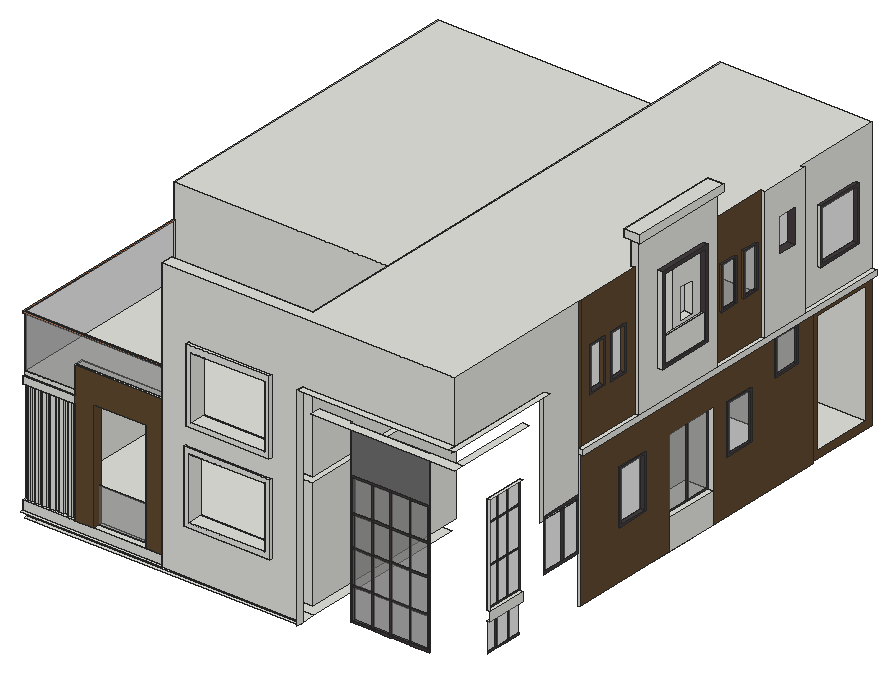
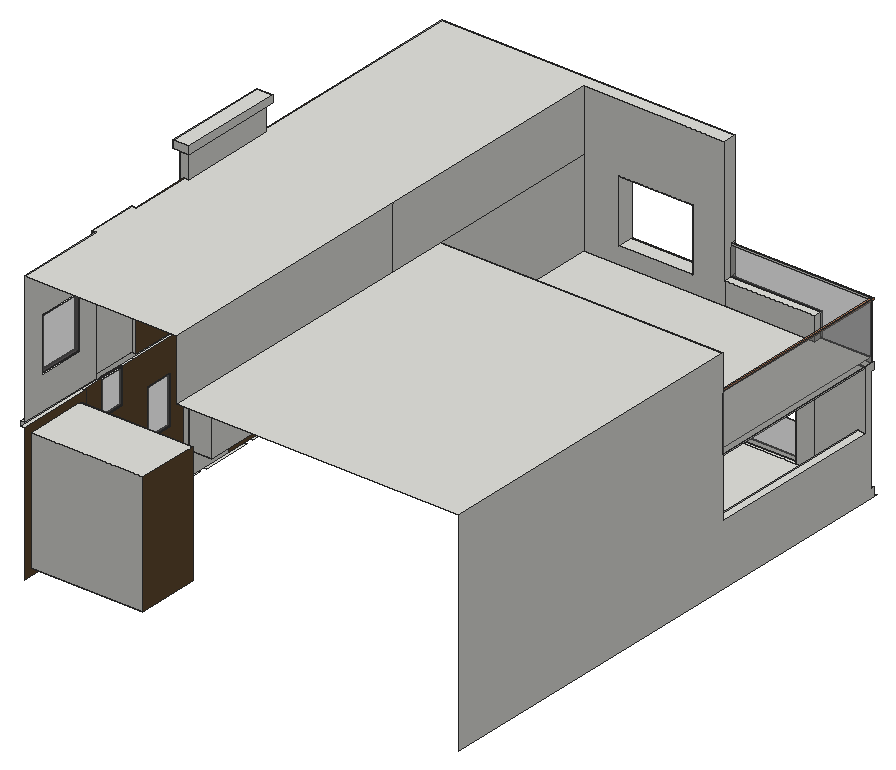
# SketchUp Ruby script. Lengths in inches.
U = 1.inch
M = Sketchup.active_model
def pt(a) = Geom::Point3d.new(a.map { |v| v * U })
def face(e, loops, mat)
  f = e.add_face(loops[0].map { |a| pt(a) })
  loops[1..].each { |l| e.add_face(l.map { |a| pt(a) }).erase! }
  f.material = f.back_material = mat if mat
  f
end
# faces: each face lists its corners as indices into pts; further lists are holes
def faces(e, pts, list, mat = nil) = list.each { |f| face(e, (f[0].is_a?(Array) ? f : [f]).map { |l| l.map { |i| pts[i] } }, mat) }
# xy, xz, yz: faces in a plane at the given z, y or x. An outline is a flat list of corners, or four numbers for a rectangle; further outlines are holes
def ring(l) = l.size == 4 ? [[l[0], l[1]], [l[2], l[1]], [l[2], l[3]], [l[0], l[3]]] : l.each_slice(2).to_a
def flat(e, list, mat, &to3) = list.each { |f| face(e, (f[0].is_a?(Array) ? f : [f]).map { |l| ring(l).map { |u, v| to3.(u, v) } }, mat) }
def xy(e, z, list, mat = nil) = flat(e, list, mat) { |x, y| [x, y, z] }
def xz(e, y, list, mat = nil) = flat(e, list, mat) { |x, z| [x, y, z] }
def yz(e, x, list, mat = nil) = flat(e, list, mat) { |y, z| [x, y, z] }
def lines(e, pts, list) = list.each { |a, b| e.add_line(pt(pts[a]), pt(pts[b])) }
# prism: a flat outline (further loops are holes) pulled along v
def prism(e, loops, v, mat = nil)
  f = face(e, loops, mat); d = Geom::Vector3d.new(v.map { |x| x * U })
  f.pushpull(f.normal.samedirection?(d) ? d.length : -d.length)
end
def box(e, o, s, mat = nil) = prism(e, [[o, [o[0] + s[0], o[1], o[2]], [o[0] + s[0], o[1] + s[1], o[2]], [o[0], o[1] + s[1], o[2]]]], [0, 0, s[2]], mat)
def at(x, y, z, deg = 0) = Geom::Transformation.translation(pt([x, y, z])) * Geom::Transformation.rotation(ORIGIN, Z_AXIS, deg.degrees)
def axes(o, x, y, z) = Geom::Transformation.new([*x, 0, *y, 0, *z, 0, *pt(o).to_a, 1])
def part(name) = M.definitions.add(name)
# library, detail: a bought-in or finely detailed component or shape, given as its bounding box
def library(name, o, s) = part(name).tap { |d| box(d.entities, o, s) }
def detail(e, o, s) = box(e.add_group.entities, o, s)
def put(e, d, t, mat = nil) = e.add_instance(d, t).tap { |i| i.material = mat if mat }
def group(e, t, mat = nil) = e.add_group.tap { |g| g.transformation = t; g.material = mat if mat }.entities
root = M.entities
M.materials.add("Niraj_Hair_Dark").color = [109, 109, 109]
M.materials.add("Niraj_Shoe_Sole").color = [96, 73, 48]
M.materials.add("[Asphalt New]").color = [67, 60, 62]
M.materials.add("[Translucent Glass Gray]").color = [128, 128, 128]
M.materials["[Translucent Glass Gray]"].alpha = 0.5
M.materials.add("[Wood Veneer 02]").color = [190, 128, 91]
xy(root,1516.31,[[1247.13,2185.52,1302.24,2203.14],[1302.24,2185.52,2665.6,2203.14]])
xy(root,1537,[[1226.44,2185.52,1956.37,2203.14],[1956.37,2185.52,1956.37,2203.14,1302.24,2203.14,1302.24,2260.63,2686.29,2260.63,2686.29,2185.52],[1226.44,2203.14,1302.24,2260.63],[1226.44,2260.63,2686.29,3149.5625]])
xy(root,1540.5,[[3472.07,2984.77,3483.14,3408.39],[3467.64,3450.16,3483.14,3710.59],[3472.07,3749.47,3483.14,4486.23]])
xy(root,1579.37,[[2891.32,4525.1,3472.07,4845.12]])
xy(root,1582.55,[[1226.44,2203.14,1493.57,2203.14,1493.57,2218.08,1483.28,2218.08,1483.28,2223.46,1465.16,2223.46,1465.16,2218.08,1446.59,2218.08,1446.59,2223.46,1424.59,2223.46,1424.59,2218.08,1399.61,2218.08,1399.61,2223.46,1381.49,2223.46,1381.49,2218.08,1354.55,2218.08,1354.55,2223.46,1336.43,2223.46,1336.43,2218.08,1313.55,2218.08,1313.55,2223.46,1295.43,2223.46,1295.43,2218.08,1274.36,2218.08,1274.36,2223.46,1256.24,2223.46,1256.24,2218.08,1238.78,2218.08,1238.78,2223.46,1226.44,2223.46],[1591.04,2203.14,1861.04,2235.67],[1591.04,2236.36,1861.04,2252.19],[1270.45,2252.19,2686.29,3178.12]])
xy(root,1627.62,[[2937.39,2198.52,3320.92,2205.96]],"[Asphalt New]")
xy(root,1695.84,[[3331.64,3559.17,3452.14,3848.98],[3452.14,3559.17,3483.14,3848.98]])
xy(root,1704.14,[[3452.14,3567.47,3454.7,3840.68]],"[Asphalt New]")
xy(root,1715.07,[[3456.14,2414.23,3472.07,2625.31]])
xy(root,1763.16,[[3456.14,2414.23,3472.07,2625.31]])
xy(root,1766.92,[[1591.04,2235.67,1861.04,2236.36]])
xy(root,1776.43,[[2083.24,2174.39,2526.93,2185.52]])
xy(root,1801.58,[[2108.4,2174.39,2501.77,2252.19]])
xy(root,1802.3,[[3483.14,3228.05,3492.07,3398.55]],"[Asphalt New]")
xy(root,1809.31,[[3472.07,3235.0625,3492.07,3391.54]],"[Asphalt New]")
xy(root,1822.36,[[3483.14,3924.38,3494.39,4081.63]])
xy(root,1829.25,[[3483.14,3931.27,3494.39,4074.74]],"[Asphalt New]")
xy(root,1849.86,[[1226.44,2252.19,1270.45,3178.12]])
xy(root,2054.62,[[3483.14,4232.85,3494.39,4378.16]],"[Asphalt New]")
xy(root,2062.24,[[3483.14,4240.47,3494.39,4370.54]],"[Asphalt New]")
xy(root,2069.91,[[3483.14,3931.27,3494.39,4074.74]])
xy(root,2071.16,[[3472.07,3235.0625,3492.07,3391.54]])
xy(root,2076.35,[[3452.14,3567.47,3454.7,3840.68]],"[Asphalt New]")
xy(root,2076.8,[[3483.14,3924.38,3494.39,4081.63]],"[Asphalt New]")
xy(root,2078.17,[[3483.14,3228.05,3492.07,3398.55]],"[Asphalt New]")
xy(root,2084.65,[[3331.64,3559.17,3452.14,3848.98],[3452.14,3559.17,3483.14,3848.98]])
xy(root,2121.39,[[2108.4,2174.39,2501.77,2252.19]])
xy(root,2123.54,[[1226.44,2203.14,1226.44,2223.46,1238.78,2223.46,1238.78,2218.08,1256.24,2218.08,1256.24,2223.46,1274.36,2223.46,1274.36,2218.08,1295.43,2218.08,1295.43,2223.46,1313.55,2223.46,1313.55,2218.08,1336.43,2218.08,1336.43,2223.46,1354.55,2223.46,1354.55,2218.08,1381.49,2218.08,1381.49,2223.46,1399.61,2223.46,1399.61,2218.08,1424.59,2218.08,1424.59,2223.46,1446.59,2223.46,1446.59,2218.08,1465.16,2218.08,1465.16,2223.46,1483.28,2223.46,1483.28,2218.08,1493.57,2218.08,1493.57,2203.14]])
xy(root,2146.55,[[2083.24,2174.39,2526.93,2185.52]])
xy(root,2152.61,[[1591.04,2203.14,1861.04,2252.19]])
xy(root,2155.05,[[1226.44,2252.19,2686.29,3178.12]])
xy(root,2159.11,[[1226.44,2203.14,1493.57,2211.6],[1226.44,2211.6,1493.57,2252.19]])
xy(root,2182.99,[[1235.99,2211.6,1493.57,2211.6,1493.57,2252.19,2686.29,2252.19,2686.29,3178.12,1235.99,3178.12]])
xy(root,2203.625,[[2891.32,4525.1,3472.07,4845.12]])
xy(root,2234.875,[[3483.14,4240.47,3494.39,4370.54]])
xy(root,2242.5,[[3483.14,2984.77,3494.39,4163.67],[3483.14,4163.67,3494.39,4232.85],[3483.14,4378.16,3494.39,4486.23],[3472.07,4486.23,3494.39,4883.98]])
xy(root,2245.25,[[2096.43,2168.96,2526.93,2185.52]])
xy(root,2269.31,[[3472.07,2984.77,3494.39,3350.15],[3472.07,3853.15,3494.39,4163.67],[3472.07,4422.53,3494.39,4883.98]])
xy(root,2269.67,[[2120.84,2168.96,2502.51,2252.19]])
xy(root,2280.66,[[3456.14,2414.23,3472.07,2625.31]])
xy(root,2289.375,[[2937.39,2198.52,3320.92,2205.96]],"[Asphalt New]")
xy(root,2302.92,[[1493.57,2203.14,1956.37,2211.6],[1493.57,2211.6,1956.37,2252.19]])
xy(root,2436.24,[[3472.07,4525.34,3492.2,4774.84]])
xy(root,2437.0625,[[3494.39,3467.06,3522.14,3759.64]])
xy(root,2447.05,[[3472.07,4536.15,3492.2,4764.03]],"[Asphalt New]")
xy(root,2449.71,[[1226.44,2203.14,1956.37,2211.6]])
xy(root,2452.01,[[3435.7,3482.01,3504.09,3482.01,3504.09,3744.69,3494.39,3744.69,3494.39,3569.97,3435.7,3569.97]])
xy(root,2452.01,[[3512.34,3482.01,3522.14,3744.69]],"[Asphalt New]")
xy(root,2457.42,[[1226.44,2203.14,1956.37,2203.14,1956.37,2211.6,1235.99,2211.6,1235.99,3178.12,1226.44,3178.12]],"[Wood Veneer 02]")
xy(root,2488.0625,[[3472.07,3188.64,3478.64,3285.58]],"Niraj_Shoe_Sole")
xy(root,2490.9375,[[3472.07,3051.47,3478.64,3149.03]],"Niraj_Shoe_Sole")
xy(root,2494.75,[[3459.7,3195.33,3478.64,3278.89]],"[Asphalt New]")
xy(root,2497.43,[[3459.7,3057.97,3478.64,3142.54]],"[Asphalt New]")
xy(root,2501.88,[[3472.07,4037.52,3485.45,4130.96]],"Niraj_Shoe_Sole")
xy(root,2502.51,[[3472.07,3896.77,3485.45,3993.33]],"Niraj_Shoe_Sole")
xy(root,2507.66,[[3472.07,4043.3,3485.45,4125.18]],"[Asphalt New]")
xy(root,2508.3,[[3472.07,3902.5625,3485.45,3987.53]],"[Asphalt New]")
xy(root,2542.29,[[2759.375,2150.08,2759.375,2203.14,2926.88,2203.14,2926.88,2198.52,3331.43,2198.52,3331.43,2203.14,3502.39,2203.14,3502.39,2150.08],[3472.07,2203.14,3502.39,2625.31]])
xy(root,2576.14,[[3504.09,3482.01,3512.34,3744.69]])
xy(root,2587.3125,[[3454.07,3612.98,3494.39,3696.29]])
xy(root,2596.53,[[2120.84,2168.96,2502.51,2252.19]])
xy(root,2613.09,[[3451.2,4253.76,3494.39,4365.63]],"[Asphalt New]")
xy(root,2628.8125,[[2686.29,2150.08,3472.07,2185.52],[3472.07,2150.08,3502.39,2760.56],[2096.43,2168.96,2526.93,2185.52],[1226.44,3178.12,2686.29,4883.98]])
xy(root,2709.86,[[3472.07,4536.15,3492.2,4764.03]])
xy(root,2713.875,[[3459.7,3195.33,3478.64,3278.89]],"Niraj_Shoe_Sole")
xy(root,2714.07,[[3459.7,3057.97,3478.64,3142.54]],"Niraj_Shoe_Sole")
xy(root,2718.09,[[3472.07,3902.5625,3485.45,3987.53]],"Niraj_Shoe_Sole")
xy(root,2718.11,[[3472.07,4043.3,3485.45,4125.18]],"Niraj_Shoe_Sole")
xy(root,2720.5625,[[3472.07,3051.47,3478.64,3149.03],[3472.07,3188.64,3478.64,3285.58]],"[Asphalt New]")
xy(root,2720.68,[[3472.07,4525.34,3492.2,4774.84]],"[Asphalt New]")
xy(root,2723.88,[[3472.07,3896.77,3485.45,3993.33],[3472.07,4037.52,3485.45,4130.96]],"[Asphalt New]")
xy(root,2746.375,[[3454.07,3612.98,3494.39,3696.29]])
xy(root,2792.84,[[3451.2,4253.76,3494.39,4365.63]],"[Asphalt New]")
xy(root,2877.05,[[3435.7,3482.01,3435.7,3569.97,3494.39,3569.97,3494.39,3744.69,3522.14,3744.69,3522.14,3482.01]])
xy(root,2892,[[3494.39,3467.06,3522.14,3759.64]],"[Asphalt New]")
xy(root,2946.875,[[1956.37,2185.52,3472.07,2185.52,3472.07,3350.15,3449.89,3350.15,3449.89,3853.15,3472.07,3853.15,3472.07,4163.67,3494.39,4163.67,3494.39,4422.53,3472.07,4422.53,3472.07,4883.98,2686.29,4883.98,2686.29,2252.19,1956.37,2252.19]])
xy(root,3079.5,[[[3430.47,3330.74,3513.81,3872.56],[3449.89,3350.15,3494.39,3853.15]]])
xy(root,3117.8125,[[3430.47,3330.74,3513.81,3872.56]])
xz(root,2168.96,[[[2096.43,2245.25,2526.93,2628.8125],[2120.84,2269.67,2502.51,2596.53]]])
xz(root,2174.39,[[[2083.24,1776.43,2526.93,2146.55],[2108.4,1801.58,2501.77,2121.39]]])
xz(root,2185.52,[[[1956.37,1537,2686.29,1537,2686.29,2628.8125,3472.07,2628.8125,3472.07,2946.875,1956.37,2946.875],[2096.43,2245.25,2526.93,2628.8125],[2083.24,1776.43,2526.93,2146.55]]])
xz(root,2198.52,[[2926.88,2299.88,3331.43,2542.29]],"Niraj_Hair_Dark")
xz(root,2198.52,[[2926.88,1617.11,3033.28,1617.11,3033.28,1627.62,2937.39,1627.62,2937.39,2289.375,3129.16,2289.375,3129.16,2299.88,2926.88,2299.88],[3033.28,1617.11,3041.55,1627.62],[3041.55,1617.11,3129.16,1627.62],[3129.16,1617.11,3135.04,1627.62],[3135.04,1617.11,3227.98,1627.62],
  [3236.17,1617.11,3331.43,1617.11,3331.43,2299.88,3135.04,2299.88,3135.04,2289.375,3320.92,2289.375,3320.92,1627.62,3236.17,1627.62],[3227.98,1617.11,3236.17,1627.62],[3033.28,1627.62,3041.55,1784.53],[3129.16,1627.62,3135.04,1784.53],[3227.98,1627.62,3236.17,1784.53],
  [2937.39,1784.53,3033.28,1793.06],[3033.28,1784.53,3041.55,1793.06],[3041.55,1784.53,3129.16,1793.06],[3129.16,1784.53,3135.04,1793.06],[3135.04,1784.53,3227.98,1793.06],
  [3227.98,1784.53,3236.17,1793.06],[3236.17,1784.53,3320.92,1793.06],[3033.28,1793.06,3041.55,1958.49],[3129.16,1793.06,3135.04,1958.49],[3227.98,1793.06,3236.17,1958.49],
  [2937.39,1958.49,3033.28,1968.01],[3033.28,1958.49,3041.55,1968.01],[3041.55,1958.49,3129.16,1968.01],[3129.16,1958.49,3135.04,1968.01],[3135.04,1958.49,3227.98,1968.01],
  [3227.98,1958.49,3236.17,1968.01],[3236.17,1958.49,3320.92,1968.01],[3033.28,1968.01,3041.55,2119.24],[3129.16,1968.01,3135.04,2119.24],[3227.98,1968.01,3236.17,2119.24],
  [2937.39,2119.24,3033.28,2128.69],[3033.28,2119.24,3041.55,2128.69],[3041.55,2119.24,3129.16,2128.69],[3129.16,2119.24,3135.04,2128.69],[3135.04,2119.24,3227.98,2128.69],
  [3227.98,2119.24,3236.17,2128.69],[3236.17,2119.24,3320.92,2128.69],[3033.28,2128.69,3041.55,2289.375],[3129.16,2128.69,3135.04,2289.375],[3227.98,2128.69,3236.17,2289.375],
  [3129.16,2289.375,3135.04,2299.88]],"[Asphalt New]")
xz(root,2198.52,[[2937.39,1627.62,3033.28,1784.53],[3041.55,1627.62,3129.16,1784.53],[3135.04,1627.62,3227.98,1784.53],[3236.17,1627.62,3320.92,1784.53],[2937.39,1793.06,3033.28,1958.49],
  [3041.55,1793.06,3129.16,1958.49],[3135.04,1793.06,3227.98,1958.49],[3236.17,1793.06,3320.92,1958.49],[2937.39,1968.01,3033.28,2119.24],[3041.55,1968.01,3129.16,2119.24],
  [3135.04,1968.01,3227.98,2119.24],[3236.17,1968.01,3320.92,2119.24],[2937.39,2128.69,3033.28,2289.375],[3041.55,2128.69,3129.16,2289.375],[3135.04,2128.69,3227.98,2289.375],
  [3236.17,2128.69,3320.92,2289.375]],"[Translucent Glass Gray]")
xz(root,2203.14,[[1226.44,1537,1956.37,1582.55],[1226.44,2123.54,1493.57,2159.11]])
xz(root,2203.14,[[1493.57,1582.55,1591.04,1582.55,1591.04,2152.61,1861.04,2152.61,1861.04,1582.55,1956.37,1582.55,1956.37,2302.92,1493.57,2302.92]],"Niraj_Shoe_Sole")
xz(root,2203.14,[[1226.44,2449.71,1956.37,2457.42]],"[Wood Veneer 02]")
xz(root,2205.96,[[2937.39,1627.62,3320.92,2289.375]],"[Translucent Glass Gray]")
xz(root,2211.6,[[1226.44,2159.11,1493.57,2159.11,1493.57,2182.99,1235.99,2182.99,1235.99,2449.71,1226.44,2449.71],[1235.99,2449.71,1956.37,2457.42]])
xz(root,2211.6,[[1235.99,2182.99,1235.99,2449.71,1956.37,2449.71,1956.37,2302.92,1493.57,2302.92,1493.57,2182.99]],"[Translucent Glass Gray]")
xz(root,2218.08,[[1238.78,1582.55,1256.24,2123.54],[1274.36,1582.55,1295.43,2123.54],[1313.55,1582.55,1336.43,2123.54],[1354.55,1582.55,1381.49,2123.54],[1399.61,1582.55,1424.59,2123.54],
  [1446.59,1582.55,1465.16,2123.54],[1483.28,1582.55,1493.57,2123.54]])
xz(root,2223.46,[[1226.44,1582.55,1238.78,2123.54],[1256.24,1582.55,1274.36,2123.54],[1295.43,1582.55,1313.55,2123.54],[1336.43,1582.55,1354.55,2123.54],[1381.49,1582.55,1399.61,2123.54],
  [1424.59,1582.55,1446.59,2123.54],[1465.16,1582.55,1483.28,2123.54]])
xz(root,2236.36,[[1591.04,1582.55,1861.04,1766.92]],"[Translucent Glass Gray]")
xz(root,2252.19,[[1270.45,1582.55,1270.45,1849.86,1226.44,1849.86,1226.44,2155.05,1493.57,2155.05,1493.57,1582.55],[1493.57,1582.55,1591.04,2155.05],[1861.04,1582.55,1956.37,2155.05],[[1956.37,1582.55,2686.29,2155.05],[2108.4,1801.58,2501.77,2121.39]],[1591.04,2152.61,1861.04,2155.05],
  [1226.44,2155.05,1493.57,2159.11],[1493.57,2182.99,1956.37,2302.92],[[1956.37,2182.99,2686.29,2946.875],[2120.84,2269.67,2502.51,2596.53]]])
xz(root,2414.23,[[3456.14,1763.16,3472.07,2280.66]])
xz(root,2984.77,[[3472.07,1540.5,3483.14,2242.5],[3472.07,2242.5,3494.39,2269.31]])
xz(root,3051.47,[[3472.07,2490.9375,3478.64,2720.5625]],"Niraj_Shoe_Sole")
xz(root,3057.97,[[3459.7,2497.43,3478.64,2714.07]],"Niraj_Shoe_Sole")
xz(root,3142.54,[[3459.7,2497.43,3478.64,2714.07]],"Niraj_Shoe_Sole")
xz(root,3149.03,[[3472.07,2490.9375,3478.64,2720.5625]],"Niraj_Shoe_Sole")
xz(root,3178.12,[[1270.45,1582.55,2686.29,1582.55,2686.29,2155.05,1226.44,2155.05,1226.44,1849.86,1270.45,1849.86],[1235.99,2182.99,2686.29,2182.99,2686.29,2628.8125,1226.44,2628.8125,1226.44,2457.42,1235.99,2457.42]])
xz(root,3188.64,[[3472.07,2488.0625,3478.64,2720.5625]],"Niraj_Shoe_Sole")
xz(root,3195.33,[[3459.7,2494.75,3478.64,2713.875]],"Niraj_Shoe_Sole")
xz(root,3228.05,[[3483.14,1802.3,3492.07,2078.17]],"[Asphalt New]")
xz(root,3235.0625,[[3472.07,1809.31,3492.07,2071.16]])
xz(root,3278.89,[[3459.7,2494.75,3478.64,2713.875]],"Niraj_Shoe_Sole")
xz(root,3285.58,[[3472.07,2488.0625,3478.64,2720.5625]],"Niraj_Shoe_Sole")
xz(root,3330.74,[[3430.47,3079.5,3513.81,3117.8125]])
xz(root,3350.15,[[3472.07,2269.31,3494.39,2269.31,3494.39,3079.5,3449.89,3079.5,3449.89,2946.875,3472.07,2946.875]])
xz(root,3391.54,[[3472.07,1809.31,3492.07,2071.16]],"[Asphalt New]")
xz(root,3398.55,[[3483.14,1802.3,3492.07,2078.17]],"[Asphalt New]")
xz(root,3467.06,[[3494.39,2437.0625,3522.14,2892]])
xz(root,3482.01,[[3435.7,2452.01,3435.7,2877.05,3522.14,2877.05,3522.14,2452.01,3512.34,2452.01,3512.34,2576.14,3504.09,2576.14,3504.09,2452.01]],"[Asphalt New]")
xz(root,3559.17,[[3331.64,1695.84,3452.14,2084.65],[3452.14,1695.84,3483.14,2084.65]])
xz(root,3567.47,[[3452.14,1704.14,3454.7,2076.35]],"[Asphalt New]")
xz(root,3569.97,[[3435.7,2452.01,3494.39,2877.05]])
xz(root,3612.98,[[3454.07,2587.3125,3494.39,2746.375]])
xz(root,3696.29,[[3454.07,2587.3125,3494.39,2746.375]])
xz(root,3744.69,[[3494.39,2452.01,3504.09,2452.01,3504.09,2576.14,3512.34,2576.14,3512.34,2452.01,3522.14,2452.01,3522.14,2877.05,3494.39,2877.05]],"[Asphalt New]")
xz(root,3759.64,[[3494.39,2437.0625,3522.14,2892]])
xz(root,3840.68,[[3452.14,1704.14,3454.7,2076.35]],"[Asphalt New]")
xz(root,3848.98,[[3331.64,1695.84,3452.14,2084.65],[3452.14,1695.84,3483.14,2084.65]])
xz(root,3853.15,[[3472.07,2269.31,3472.07,2946.875,3449.89,2946.875,3449.89,3079.5,3494.39,3079.5,3494.39,2269.31]])
xz(root,3872.56,[[3430.47,3079.5,3513.81,3117.8125]])
xz(root,3896.77,[[3472.07,2502.51,3485.45,2723.88]],"Niraj_Shoe_Sole")
xz(root,3902.5625,[[3472.07,2508.3,3485.45,2718.09]],"Niraj_Shoe_Sole")
xz(root,3924.38,[[3483.14,1822.36,3494.39,2076.8]],"[Asphalt New]")
xz(root,3931.27,[[3483.14,1829.25,3494.39,2069.91]],"[Asphalt New]")
xz(root,3987.53,[[3472.07,2508.3,3485.45,2718.09]],"Niraj_Shoe_Sole")
xz(root,3993.33,[[3472.07,2502.51,3485.45,2723.88]],"Niraj_Shoe_Sole")
xz(root,4037.52,[[3472.07,2501.88,3485.45,2723.88]],"Niraj_Shoe_Sole")
xz(root,4043.3,[[3472.07,2507.66,3485.45,2718.11]],"Niraj_Shoe_Sole")
xz(root,4074.74,[[3483.14,1829.25,3494.39,2069.91]],"[Asphalt New]")
xz(root,4081.63,[[3483.14,1822.36,3494.39,2076.8]])
xz(root,4125.18,[[3472.07,2507.66,3485.45,2718.11]],"Niraj_Shoe_Sole")
xz(root,4130.96,[[3472.07,2501.88,3485.45,2723.88]],"Niraj_Shoe_Sole")
xz(root,4163.67,[[3472.07,2269.31,3494.39,2946.875]])
xz(root,4232.85,[[3483.14,2054.62,3494.39,2242.5]],"[Asphalt New]")
xz(root,4240.47,[[3483.14,2062.24,3494.39,2234.875]])
xz(root,4253.76,[[3451.2,2613.09,3494.39,2792.84]],"[Asphalt New]")
xz(root,4365.63,[[3451.2,2613.09,3494.39,2792.84]],"[Asphalt New]")
xz(root,4370.54,[[3483.14,2062.24,3494.39,2234.875]],"[Asphalt New]")
xz(root,4378.16,[[3483.14,2054.62,3494.39,2242.5]],"[Asphalt New]")
xz(root,4422.53,[[3472.07,2269.31,3494.39,2946.875]])
xz(root,4486.23,[[3472.07,1540.5,3483.14,2242.5]])
xz(root,4525.1,[[2891.32,1579.37,3472.07,2203.625]])
xz(root,4525.34,[[3472.07,2436.24,3492.2,2720.68]])
xz(root,4536.15,[[3472.07,2447.05,3492.2,2709.86]],"[Asphalt New]")
xz(root,4764.03,[[3472.07,2447.05,3492.2,2709.86]],"[Asphalt New]")
xz(root,4774.84,[[3472.07,2436.24,3492.2,2720.68]])
xz(root,4845.12,[[2891.32,1579.37,3472.07,2203.625]])
yz(root,1226.44,[[2203.14,1537,2203.14,1582.55,2223.46,1582.55,2223.46,2123.54,2203.14,2123.54,2203.14,2159.11,2252.19,2159.11,2252.19,1849.86,3178.12,1849.86,3178.12,2628.8125,4883.98,2628.8125,4883.98,1537],[2252.19,2155.05,3178.12,2159.11]])
yz(root,1226.44,[[2211.6,2159.11,3178.12,2449.71]],"[Translucent Glass Gray]")
yz(root,1226.44,[[2203.14,2449.71,3178.12,2457.42]],"[Wood Veneer 02]")
yz(root,1238.78,[[2218.08,1582.55,2223.46,2123.54]])
yz(root,1256.24,[[2218.08,1582.55,2223.46,2123.54]])
yz(root,1270.45,[[2252.19,1582.55,3178.12,1849.86]])
yz(root,1274.36,[[2218.08,1582.55,2223.46,2123.54]])
yz(root,1295.43,[[2218.08,1582.55,2223.46,2123.54]])
yz(root,1313.55,[[2218.08,1582.55,2223.46,2123.54]])
yz(root,1336.43,[[2218.08,1582.55,2223.46,2123.54]])
yz(root,1354.55,[[2218.08,1582.55,2223.46,2123.54]])
yz(root,1381.49,[[2218.08,1582.55,2223.46,2123.54]])
yz(root,1399.61,[[2218.08,1582.55,2223.46,2123.54]])
yz(root,1424.59,[[2218.08,1582.55,2223.46,2123.54]])
yz(root,1446.59,[[2218.08,1582.55,2223.46,2123.54]])
yz(root,1465.16,[[2218.08,1582.55,2223.46,2123.54]])
yz(root,1483.28,[[2218.08,1582.55,2223.46,2123.54]])
yz(root,1493.57,[[2203.14,1582.55,2218.08,2123.54],[2203.14,2159.11,2211.6,2182.99],[2203.14,2182.99,2211.6,2302.92],[2211.6,2182.99,2252.19,2302.92]])
yz(root,1591.04,[[2203.14,1582.55,2235.67,1582.55,2235.67,1766.92,2236.36,1766.92,2236.36,1582.55,2252.19,1582.55,2252.19,2152.61,2203.14,2152.61]],"Niraj_Shoe_Sole")
yz(root,1861.04,[[2203.14,1582.55,2203.14,2152.61,2252.19,2152.61,2252.19,1582.55,2236.36,1582.55,2236.36,1766.92,2235.67,1766.92,2235.67,1582.55]],"Niraj_Shoe_Sole")
yz(root,1956.37,[[2185.52,1537,2203.14,1582.55],[2185.52,1582.55,2203.14,2302.92],[2185.52,2302.92,2211.6,2449.71],[2211.6,2302.92,2211.6,2457.42,2185.52,2457.42,2185.52,2946.875,2252.19,2946.875,2252.19,2302.92],[2185.52,2449.71,2203.14,2457.42]])
yz(root,2083.24,[[2174.39,1776.43,2185.52,2146.55]])
yz(root,2096.43,[[2168.96,2245.25,2185.52,2628.8125]])
yz(root,2108.4,[[2174.39,1801.58,2252.19,2121.39]])
yz(root,2120.84,[[2168.96,2269.67,2252.19,2596.53]])
yz(root,2501.77,[[2174.39,1801.58,2252.19,2121.39]])
yz(root,2502.51,[[2168.96,2269.67,2252.19,2596.53]])
yz(root,2526.93,[[2174.39,1776.43,2185.52,2146.55],[2168.96,2245.25,2185.52,2628.8125]])
yz(root,2686.29,[[2150.08,1537,2185.52,2628.8125],[2252.19,1582.55,3178.12,2155.05],[2252.19,2182.99,3178.12,2628.8125],[2252.19,2628.8125,3487.33,2946.875],[3487.33,2628.8125,4883.98,2946.875]])
yz(root,2891.32,[[4525.1,1579.37,4845.12,2203.625]],"Niraj_Shoe_Sole")
yz(root,2926.88,[[2198.52,2299.88,2203.14,2542.29]],"Niraj_Hair_Dark")
yz(root,2926.88,[[2198.52,1617.11,2203.14,2299.88]],"[Asphalt New]")
yz(root,2937.39,[[2198.52,1627.62,2205.96,2289.375]],"[Asphalt New]")
yz(root,3320.92,[[2198.52,1627.62,2205.96,2289.375]],"[Asphalt New]")
yz(root,3331.43,[[2198.52,2299.88,2203.14,2542.29]],"Niraj_Hair_Dark")
yz(root,3331.43,[[2198.52,1617.11,2203.14,2299.88]],"[Asphalt New]")
yz(root,3331.64,[[3559.17,1695.84,3848.98,2084.65]])
yz(root,3430.47,[[3330.74,3079.5,3872.56,3117.8125]])
yz(root,3435.7,[[3482.01,2452.01,3569.97,2877.05]])
yz(root,3449.89,[[3350.15,2946.875,3853.15,3079.5]])
yz(root,3451.2,[[4253.76,2613.09,4365.63,2792.84]],"[Translucent Glass Gray]")
yz(root,3452.14,[[[3559.17,1695.84,3848.98,2084.65],[3567.47,1704.14,3840.68,2076.35]]],"[Asphalt New]")
yz(root,3454.07,[[[3611.68,2586.01,3697.59,2747.68],[3612.98,2587.3125,3696.29,2746.375]],[3612.98,2587.3125,3696.29,2746.375]],"[Translucent Glass Gray]")
yz(root,3454.7,[[3704.08,1704.14,3713.65,2076.35]],"[Asphalt New]")
yz(root,3454.7,[[3567.47,1704.14,3704.08,2076.35],[3713.65,1704.14,3840.68,2076.35]],"[Translucent Glass Gray]")
yz(root,3456.14,[[2420.15,1560.48,2466.95,1568.08],[2466.95,1560.48,2475.41,1568.08],[2475.41,1560.48,2547.4,1568.08],[2547.4,1560.48,2555.61,1568.08],[2555.61,1560.48,2619.39,1568.08],
  [2466.95,1568.08,2475.41,1709.15],[2547.4,1568.08,2555.61,1709.15],[[2414.23,1763.16,2625.31,2280.66],[2420.47,1769.4,2619.07,2274.42]],[2477.71,1769.4,2483.88,1957.67],[2543.97,1769.4,2550.82,1957.67],
  [2420.47,1957.67,2477.71,1963.77],[2477.71,1957.67,2483.88,1963.77],[2483.88,1957.67,2543.97,1963.77],[2543.97,1957.67,2550.82,1963.77],[2550.82,1957.67,2619.07,1963.77],
  [2477.71,1963.77,2483.88,2158.15],[2543.97,1963.77,2550.82,2158.15],[2420.47,2158.15,2477.71,2163.81],[2477.71,2158.15,2483.88,2163.81],[2483.88,2158.15,2543.97,2163.81],
  [2543.97,2158.15,2550.82,2163.81],[2550.82,2158.15,2619.07,2163.81],[2477.71,2163.81,2483.88,2274.42],[2543.97,2163.81,2550.82,2274.42]],"[Asphalt New]")
yz(root,3456.14,[[2420.15,1568.08,2466.95,1709.15],[2475.41,1568.08,2547.4,1709.15],[2555.61,1568.08,2619.39,1709.15],[2420.47,1769.4,2477.71,1957.67],[2483.88,1769.4,2543.97,1957.67],
  [2550.82,1769.4,2619.07,1957.67],[2420.47,1963.77,2477.71,2158.15],[2483.88,1963.77,2543.97,2158.15],[2550.82,1963.77,2619.07,2158.15],[2420.47,2163.81,2477.71,2274.42],
  [2483.88,2163.81,2543.97,2274.42],[2550.82,2163.81,2619.07,2274.42]],"[Translucent Glass Gray]")
yz(root,3459.7,[[3195.33,2494.75,3278.89,2713.875],[3057.97,2497.43,3142.54,2714.07]],"[Translucent Glass Gray]")
yz(root,3472.07,[[2414.23,1715.07,2625.31,1763.16],[2739.63,2029.65,2760.56,2029.65,2760.56,2628.8125,2164.59,2628.8125,2164.59,2607.89,2739.63,2607.89],[2984.77,2029.65,3005.69,2269.31],[2760.56,2050.57,2984.77,2050.57,2984.77,2946.875,2185.52,2946.875,2185.52,2628.8125,2760.56,2628.8125],[[4422.53,2269.31,4883.98,2946.875],[4525.34,2436.24,4774.84,2720.68]]])
yz(root,3472.07,[[[4486.23,1540.5,4883.98,2242.5],[4525.1,1579.37,4845.12,2203.625]],[2984.77,2269.31,3005.69,2946.875],[[3005.69,2269.31,3350.15,2946.875],[3188.64,2488.0625,3285.58,2720.5625],[3051.47,2490.9375,3149.03,2720.5625]],[[3853.15,2269.31,4163.67,2946.875],[3896.77,2502.51,3993.33,2723.88],[4037.52,2501.88,4130.96,2723.88]]],"Niraj_Shoe_Sole")
yz(root,3472.07,[[2760.56,1781.04,2984.77,1781.04,2984.77,2029.65,2973.27,2029.65,2973.27,1792.53,2772.05,1792.53,2772.05,2029.65,2760.56,2029.65],[2872.66,1792.53,2889.8,2029.65],[2760.56,2029.65,2772.05,2029.65,2772.05,2039.08,2973.27,2039.08,2973.27,2029.65,2984.77,2029.65,2984.77,2050.57,2760.56,2050.57],[2872.66,2029.65,2889.8,2039.08]],"[Asphalt New]")
yz(root,3472.07,[[2772.05,1792.53,2872.66,2029.65],[2889.8,1792.53,2973.27,2029.65],[3235.0625,1809.31,3391.54,2071.16],[2772.05,2029.65,2872.66,2039.08],[2889.8,2029.65,2973.27,2039.08],
  [4536.15,2447.05,4764.03,2709.86],[4043.3,2507.66,4125.18,2718.11],[3902.5625,2508.3,3987.53,2718.09]],"[Translucent Glass Gray]")
yz(root,3478.64,[[[3188.64,2488.0625,3285.58,2720.5625],[3195.33,2494.75,3278.89,2713.875]],[[3051.47,2490.9375,3149.03,2720.5625],[3057.97,2497.43,3142.54,2714.07]]],"[Asphalt New]")
yz(root,3483.14,[[3559.17,1540.5,3848.98,1695.84]])
yz(root,3483.14,[[[2984.77,1540.5,3559.17,1540.5,3559.17,2084.65,3848.98,2084.65,3848.98,1540.5,4486.23,1540.5,4486.23,2242.5,4378.16,2242.5,4378.16,2054.62,4232.85,2054.62,4232.85,2242.5,2984.77,2242.5],[3228.05,1802.3,3398.55,2078.17],[3924.38,1822.36,4081.63,2076.8]]],"Niraj_Shoe_Sole")
yz(root,3483.14,[[3931.27,1829.25,4074.74,2069.91],[4240.47,2062.24,4370.54,2234.875]],"[Translucent Glass Gray]")
yz(root,3485.45,[[[4037.52,2501.88,4130.96,2723.88],[4043.3,2507.66,4125.18,2718.11]],[[3896.77,2502.51,3993.33,2723.88],[3902.5625,2508.3,3987.53,2718.09]]],"[Asphalt New]")
yz(root,3492.07,[[[3228.05,1802.3,3398.55,2078.17],[3235.0625,1809.31,3391.54,2071.16]]],"[Asphalt New]")
yz(root,3492.2,[[[4525.34,2436.24,4774.84,2720.68],[4536.15,2447.05,4764.03,2709.86]]],"[Asphalt New]")
yz(root,3494.39,[[2984.77,2242.5,4883.98,2269.31],[[3350.15,2269.31,3853.15,3079.5],[3467.06,2437.0625,3759.64,2892]],[[4163.67,2269.31,4422.53,2946.875],[4253.76,2613.09,4365.63,2792.84]],[[3569.97,2452.01,3744.69,2877.05],[3612.98,2587.3125,3696.29,2746.375]]])
yz(root,3494.39,[[[3924.38,1822.36,4081.63,2076.8],[3931.27,1829.25,4074.74,2069.91]],[[4232.85,2054.62,4378.16,2242.5],[4240.47,2062.24,4370.54,2234.875]]],"[Asphalt New]")
yz(root,3504.09,[[3482.01,2452.01,3744.69,2576.14]])
yz(root,3512.34,[[3482.01,2452.01,3744.69,2576.14]])
yz(root,3513.81,[[3330.74,3079.5,3872.56,3117.8125]])
yz(root,3522.14,[[[3467.06,2437.0625,3759.64,2892],[3482.01,2452.01,3744.69,2877.05]]],"[Asphalt New]")
p = [[3449.89,3853.15,3079.5],[3449.89,3853.15,3093.5625],[3494.39,3853.15,3079.5],[3494.39,3853.15,3093.5625],[3449.89,3350.15,3079.5],[3449.89,3350.15,3093.5625],
  [3494.39,3350.15,3079.5],[3494.39,3350.15,3093.5625]]
lines(root,p,[[0,1],[2,3],[4,5],[6,7]])
